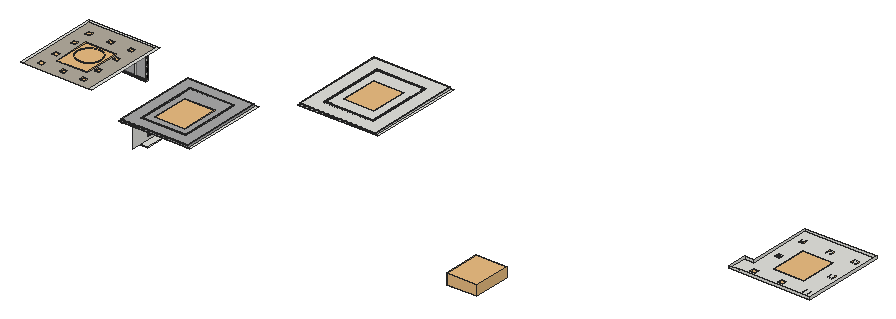
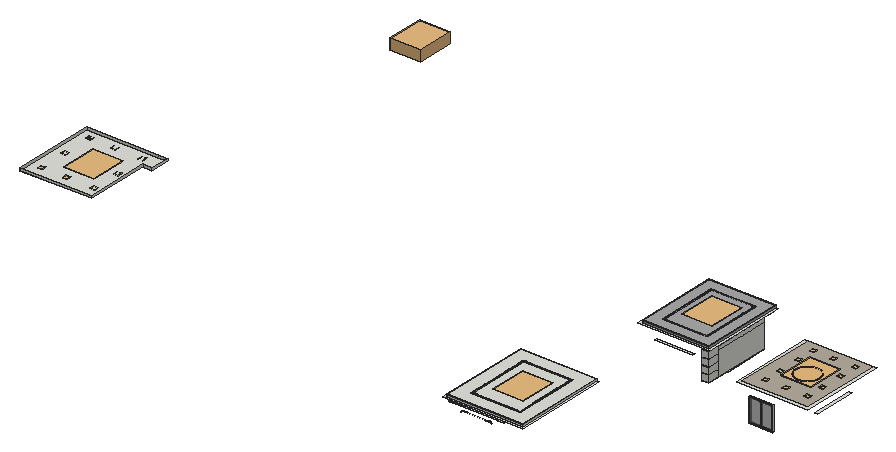
# SketchUp Ruby script. Lengths in inches.
U = 1.inch
M = Sketchup.active_model
def pt(a) = Geom::Point3d.new(a.map { |v| v * U })
def face(e, loops, mat)
  f = e.add_face(loops[0].map { |a| pt(a) })
  loops[1..].each { |l| e.add_face(l.map { |a| pt(a) }).erase! }
  f.material = f.back_material = mat if mat
  f
end
# faces: each face lists its corners as indices into pts; further lists are holes
def faces(e, pts, list, mat = nil) = list.each { |f| face(e, (f[0].is_a?(Array) ? f : [f]).map { |l| l.map { |i| pts[i] } }, mat) }
# xy, xz, yz: faces in a plane at the given z, y or x. An outline is a flat list of corners, or four numbers for a rectangle; further outlines are holes
def ring(l) = l.size == 4 ? [[l[0], l[1]], [l[2], l[1]], [l[2], l[3]], [l[0], l[3]]] : l.each_slice(2).to_a
def flat(e, list, mat, &to3) = list.each { |f| face(e, (f[0].is_a?(Array) ? f : [f]).map { |l| ring(l).map { |u, v| to3.(u, v) } }, mat) }
def xy(e, z, list, mat = nil) = flat(e, list, mat) { |x, y| [x, y, z] }
def xz(e, y, list, mat = nil) = flat(e, list, mat) { |x, z| [x, y, z] }
def yz(e, x, list, mat = nil) = flat(e, list, mat) { |y, z| [x, y, z] }
def lines(e, pts, list) = list.each { |a, b| e.add_line(pt(pts[a]), pt(pts[b])) }
# prism: a flat outline (further loops are holes) pulled along v
def prism(e, loops, v, mat = nil)
  f = face(e, loops, mat); d = Geom::Vector3d.new(v.map { |x| x * U })
  f.pushpull(f.normal.samedirection?(d) ? d.length : -d.length)
end
def box(e, o, s, mat = nil) = prism(e, [[o, [o[0] + s[0], o[1], o[2]], [o[0] + s[0], o[1] + s[1], o[2]], [o[0], o[1] + s[1], o[2]]]], [0, 0, s[2]], mat)
def at(x, y, z, deg = 0) = Geom::Transformation.translation(pt([x, y, z])) * Geom::Transformation.rotation(ORIGIN, Z_AXIS, deg.degrees)
def axes(o, x, y, z) = Geom::Transformation.new([*x, 0, *y, 0, *z, 0, *pt(o).to_a, 1])
def part(name) = M.definitions.add(name)
# library, detail: a bought-in or finely detailed component or shape, given as its bounding box
def library(name, o, s) = part(name).tap { |d| box(d.entities, o, s) }
def detail(e, o, s) = box(e.add_group.entities, o, s)
def put(e, d, t, mat = nil) = e.add_instance(d, t).tap { |i| i.material = mat if mat }
def group(e, t, mat = nil) = e.add_group.tap { |g| g.transformation = t; g.material = mat if mat }.entities
root = M.entities
M.materials.add("[0136_Charcoal]").color = [35, 35, 35]
M.materials.add("[Color M03]").color = [170, 170, 170]
M.materials.add("[Color_008]").color = [30, 30, 30]
M.materials.add("[Color_009]").color = [0, 0, 0]
M.materials.add("[Color_B19]").color = [180, 172, 158]
M.materials.add("[Translucent_Glass_Gray]").color = [128, 128, 128]
M.materials["[Translucent_Glass_Gray]"].alpha = 0.5
c1 = library("ceiling fan",[0,0,0],[76.25,93.13,30.02])
c2 = part("Enscape.LinearLight\#3")
xz(c2.entities,-55.62,[[0,-1,0,0,-0.38,-0.92],[0,-1,0.38,-0.92,0,0],[-0.38,-0.92,0,0,-0.71,-0.71],[0.38,-0.92,0.71,-0.71,0,0],[-0.71,-0.71,0,0,-0.92,-0.38],
  [0.71,-0.71,0.92,-0.38,0,0],[-0.92,-0.38,0,0,-1,0],[0.92,-0.38,1,0,0,0],[-1,0,0,0,-0.92,0.38],[0,0,-0.71,0.71,-0.92,0.38],
  [0,0,-0.38,0.92,-0.71,0.71],[0,0,0,1,-0.38,0.92],[0,0,0.38,0.92,0,1],[0,0,0.71,0.71,0.38,0.92],[0,0,0.92,0.38,0.71,0.71],
  [0,0,1,0,0.92,0.38]])
xz(c2.entities,55.62,[[0,-1,-0.38,-0.92,0,0],[0,-1,0,0,0.38,-0.92],[-0.38,-0.92,-0.71,-0.71,0,0],[0.38,-0.92,0,0,0.71,-0.71],[-0.71,-0.71,-0.92,-0.38,0,0],
  [0.71,-0.71,0,0,0.92,-0.38],[-0.92,-0.38,-1,0,0,0],[0.92,-0.38,0,0,1,0],[-1,0,-0.92,0.38,0,0],[0,0,-0.92,0.38,-0.71,0.71],
  [0,0,-0.71,0.71,-0.38,0.92],[0,0,-0.38,0.92,0,1],[0,0,0,1,0.38,0.92],[0,0,0.38,0.92,0.71,0.71],[0,0,0.71,0.71,0.92,0.38],
  [0,0,0.92,0.38,1,0]])
p = [[-0.38,-55.62,-0.92],[-0.38,55.62,-0.92],[0,55.62,-1],[0,-55.62,-1],[0.38,55.62,-0.92],[0.38,-55.62,-0.92],
  [-0.71,-55.62,-0.71],[-0.71,55.62,-0.71],[0.71,55.62,-0.71],[0.71,-55.62,-0.71],[-0.92,-55.62,-0.38],[-0.92,55.62,-0.38],
  [0.92,55.62,-0.38],[0.92,-55.62,-0.38],[-1,-55.62,0],[-1,55.62,0],[1,55.62,0],[1,-55.62,0],
  [-0.92,-55.62,0.38],[-0.92,55.62,0.38],[0.92,55.62,0.38],[0.92,-55.62,0.38],[-0.71,-55.62,0.71],[-0.71,55.62,0.71],
  [0.71,55.62,0.71],[0.71,-55.62,0.71],[-0.38,-55.62,0.92],[-0.38,55.62,0.92],[0.38,55.62,0.92],[0.38,-55.62,0.92],
  [0,-55.62,1],[0,55.62,1]]
faces(c2.entities,p,[[0,1,2],[0,2,3],[3,2,4],[3,4,5],[6,7,1],[6,1,0],[5,4,8],[5,8,9],
  [10,11,7],[10,7,6],[9,8,12],[9,12,13],[14,15,11],[14,11,10],[13,12,16],[13,16,17],
  [18,19,15],[18,15,14],[17,16,20],[17,20,21],[22,23,19],[22,19,18],[21,20,24],[21,24,25],
  [26,27,23],[26,23,22],[25,24,28],[25,28,29],[30,31,27],[30,27,26],[29,28,31],[29,31,30]])
c3 = part("Group\#24")
put(c3.entities,c2,at(55.62,1,1,-90))
put(c3.entities,c2,at(64.38,1,1,-90))
c4 = part("Group\#25")
put(c4.entities,c3,at(2,0,0,90))
put(c4.entities,c3,at(2,42,0,90))
c5 = library("Group\#26",[-1.6,-2.28,-0.2],[11.2,11.87,10.47])
c6 = library("Group\#11",[-1.89,-1.55,0],[10.94,10.95,9.68])
c7 = part("Enscape.LinearLight")
xz(c7.entities,-59.06,[[0,-1,0,0,-0.38,-0.92],[0,-1,0.38,-0.92,0,0],[-0.38,-0.92,0,0,-0.71,-0.71],[0.38,-0.92,0.71,-0.71,0,0],[-0.71,-0.71,0,0,-0.92,-0.38],
  [0.71,-0.71,0.92,-0.38,0,0],[-0.92,-0.38,0,0,-1,0],[0.92,-0.38,1,0,0,0],[-1,0,0,0,-0.92,0.38],[0,0,-0.71,0.71,-0.92,0.38],
  [0,0,-0.38,0.92,-0.71,0.71],[0,0,0,1,-0.38,0.92],[0,0,0.38,0.92,0,1],[0,0,0.71,0.71,0.38,0.92],[0,0,0.92,0.38,0.71,0.71],
  [0,0,1,0,0.92,0.38]])
xz(c7.entities,59.06,[[0,-1,-0.38,-0.92,0,0],[0,-1,0,0,0.38,-0.92],[-0.38,-0.92,-0.71,-0.71,0,0],[0.38,-0.92,0,0,0.71,-0.71],[-0.71,-0.71,-0.92,-0.38,0,0],
  [0.71,-0.71,0,0,0.92,-0.38],[-0.92,-0.38,-1,0,0,0],[0.92,-0.38,0,0,1,0],[-1,0,-0.92,0.38,0,0],[0,0,-0.92,0.38,-0.71,0.71],
  [0,0,-0.71,0.71,-0.38,0.92],[0,0,-0.38,0.92,0,1],[0,0,0,1,0.38,0.92],[0,0,0.38,0.92,0.71,0.71],[0,0,0.71,0.71,0.92,0.38],
  [0,0,0.92,0.38,1,0]])
p = [[-0.38,-59.06,-0.92],[-0.38,59.06,-0.92],[0,59.06,-1],[0,-59.06,-1],[0.38,59.06,-0.92],[0.38,-59.06,-0.92],
  [-0.71,-59.06,-0.71],[-0.71,59.06,-0.71],[0.71,59.06,-0.71],[0.71,-59.06,-0.71],[-0.92,-59.06,-0.38],[-0.92,59.06,-0.38],
  [0.92,59.06,-0.38],[0.92,-59.06,-0.38],[-1,-59.06,0],[-1,59.06,0],[1,59.06,0],[1,-59.06,0],
  [-0.92,-59.06,0.38],[-0.92,59.06,0.38],[0.92,59.06,0.38],[0.92,-59.06,0.38],[-0.71,-59.06,0.71],[-0.71,59.06,0.71],
  [0.71,59.06,0.71],[0.71,-59.06,0.71],[-0.38,-59.06,0.92],[-0.38,59.06,0.92],[0.38,59.06,0.92],[0.38,-59.06,0.92],
  [0,-59.06,1],[0,59.06,1]]
faces(c7.entities,p,[[0,1,2],[0,2,3],[3,2,4],[3,4,5],[6,7,1],[6,1,0],[5,4,8],[5,8,9],
  [10,11,7],[10,7,6],[9,8,12],[9,12,13],[14,15,11],[14,11,10],[13,12,16],[13,16,17],
  [18,19,15],[18,15,14],[17,16,20],[17,20,21],[22,23,19],[22,19,18],[21,20,24],[21,24,25],
  [26,27,23],[26,23,22],[25,24,28],[25,28,29],[30,31,27],[30,27,26],[29,28,31],[29,31,30]])
c8 = part("Group\#9")
put(c8.entities,c7,at(1,59.06,1))
put(c8.entities,c7,at(1,90.94,1))
c9 = library("Group\#10",[0,0,0],[108,2,2])
c10 = library("Group\#53",[-1.63,-0.87,0],[11.47,11.27,10.08])
c11 = library("Group\#40",[-1.73,-1.35,-0.07],[10.56,10.17,9.31])
xy(root,36,[[90,610.17,150,616.17]])
xy(root,37.6,[[555.98,931.54,615.33,932.04]])
xy(root,40,[[305.13,399.45,323.13,485.45]])
xy(root,41.5,[[305.13,518.45,323.13,546.45]])
xy(root,42,[[305.13,373.45,306.13,397.45],[306.13,397.45,323.13,487.45],[305.13,487.45,306.13,517.45]])
xy(root,42.5,[[305.13,518.45,323.13,546.45]])
xy(root,46.35,[[515.52,920.04,531.52,932.04],[637.52,920.04,653.52,932.04]])
xy(root,47.35,[[524.52,914.04,523.22,914.12,521.93,914.375,520.69,914.8,519.52,915.375,518.43,916.1,517.45,916.97,516.59,917.95,515.86,919.04,515.37,920.04,532.52,920.04,532.52,914.04],[532.52,914.04,533.52,932.04],[533.52,914.04,636.52,932.04],[636.52,914.04,636.52,920.04,653.67,920.04,653.18,919.04,652.45,917.95,651.59,916.97,650.61,916.1,649.52,915.375,648.35,914.8,647.11,914.375,645.83,914.12,644.52,914.04],[514.52,920.04,515.37,920.04,515.28,920.21,514.86,921.45,514.61,922.73,514.52,924.04],
  [653.67,920.04,654.52,920.04,654.52,924.04,654.4375,922.73,654.18,921.45,653.76,920.21]])
xy(root,51.35,[[524.52,914.04,644.52,914.04,645.83,914.12,647.11,914.375,648.35,914.8,649.52,915.375,650.61,916.1,651.59,916.97,652.45,917.95,653.18,919.04,653.76,920.21,654.18,921.45,654.4375,922.73,654.52,924.04,654.52,932.04,514.52,932.04,514.52,924.04,514.61,922.73,514.86,921.45,515.28,920.21,515.86,919.04,516.59,917.95,517.45,916.97,518.43,916.1,519.52,915.375,520.69,914.8,521.93,914.375,523.22,914.12]])
xy(root,55.35,[[462.52,698.04,468.52,698.04,468.52,932.04,660.52,932.04,660.52,698.04,666.52,698.04,666.52,938.04,462.52,938.04]])
xy(root,59.25,[[305.13,518.45,323.13,546.45]])
xy(root,60.25,[[305.13,518.45,323.13,546.45]])
xy(root,77,[[305.13,518.45,323.13,546.45]])
xy(root,78,[[305.13,518.45,323.13,546.45]])
xy(root,94.75,[[305.13,518.45,323.13,546.45]])
xy(root,95.75,[[305.13,518.45,323.13,546.45]])
xy(root,96,[[0,478.17,6,586.17],[341.13,547.45,437.13,553.45],[90,610.17,150,616.17]])
xy(root,113,[[305.13,518.45,323.13,546.45]])
xy(root,114,[[305.13,373.45,306.13,517.45],[305.13,517.45,323.13,547.45]])
xy(root,120,[[299.13,337.45,305.13,337.45,305.13,547.45,473.13,547.45,473.13,337.45,479.13,337.45,479.13,553.45,299.13,553.45],[0,400.17,6,400.17,6,610.17,174,610.17,174,400.17,180,400.17,180,616.17,0,616.17]])
xz(root,373.45,[[305.13,42,306.13,114]])
xz(root,517.45,[[306.13,42,323.13,114]])
xz(root,518.45,[[305.13,42.5,323.13,59.25],[305.13,60.25,323.13,77],[305.13,78,323.13,94.75],[305.13,95.75,323.13,113]])
xz(root,546.45,[[305.13,42.5,323.13,59.25],[305.13,60.25,323.13,77],[305.13,78,323.13,94.75],[305.13,95.75,323.13,113]])
xz(root,914.04,[[524.52,47.35,644.52,51.35]])
yz(root,90,[[610.17,36,616.17,96]])
yz(root,150,[[610.17,36,616.17,96]])
yz(root,305.13,[[518.45,42.5,546.45,59.25],[518.45,60.25,546.45,77],[518.45,78,546.45,94.75],[518.45,95.75,546.45,113]])
yz(root,306.13,[[373.45,42,517.45,102],[373.45,102,517.45,114]])
yz(root,323.13,[[518.45,41.5,546.45,42.5],[518.45,59.25,546.45,60.25],[518.45,77,546.45,78],[518.45,94.75,546.45,95.75]])
yz(root,514.52,[[924.04,47.35,932.04,51.35]])
yz(root,654.52,[[924.04,47.35,932.04,51.35]])
p = [[547.49,932.04,34.09],[546.46,932.04,32.91],[546.46,931.54,32.91],[547.49,931.54,34.09],[624.85,932.04,32.91],[623.82,932.04,34.09],
  [623.82,931.54,34.09],[624.85,931.54,32.91],[548.67,932.04,35.125],[548.67,931.54,35.125],[622.64,932.04,35.125],[622.64,931.54,35.125],
  [549.98,932.04,36],[549.98,931.54,36],[621.33,932.04,36],[621.33,931.54,36],[551.39,932.04,36.69],[551.39,931.54,36.69],
  [619.93,932.04,36.69],[619.93,931.54,36.69],[552.875,932.04,37.2],[552.875,931.54,37.2],[618.4375,932.04,37.2],[618.4375,931.54,37.2],
  [554.41,932.04,37.5],[554.41,931.54,37.5],[616.9,932.04,37.5],[616.9,931.54,37.5],[555.98,932.04,37.6],[555.98,931.54,37.6],
  [615.33,932.04,37.6],[615.33,931.54,37.6],[524.52,914.04,51.35],[523.22,914.12,51.35],[523.22,914.12,47.35],[524.52,914.04,47.35],
  [645.83,914.12,51.35],[644.52,914.04,51.35],[644.52,914.04,47.35],[645.83,914.12,47.35],[521.93,914.375,51.35],[521.93,914.375,47.35],
  [647.11,914.375,51.35],[647.11,914.375,47.35],[520.69,914.8,51.35],[520.69,914.8,47.35],[648.35,914.8,51.35],[648.35,914.8,47.35],
  [519.52,915.375,51.35],[519.52,915.375,47.35],[649.52,915.375,51.35],[649.52,915.375,47.35],[518.43,916.1,51.35],[518.43,916.1,47.35],
  [650.61,916.1,51.35],[650.61,916.1,47.35],[517.45,916.97,51.35],[517.45,916.97,47.35],[651.59,916.97,51.35],[651.59,916.97,47.35],
  [516.59,917.95,51.35],[516.59,917.95,47.35],[652.45,917.95,51.35],[652.45,917.95,47.35],[515.86,919.04,51.35],[515.86,919.04,47.35],
  [653.18,919.04,51.35],[653.18,919.04,47.35],[515.28,920.21,51.35],[515.28,920.21,47.35],[515.37,920.04,47.35],[653.76,920.21,51.35],
  [653.67,920.04,47.35],[653.76,920.21,47.35],[514.86,921.45,51.35],[514.86,921.45,47.35],[654.18,921.45,51.35],[654.18,921.45,47.35],
  [514.61,922.73,51.35],[514.61,922.73,47.35],[654.4375,922.73,51.35],[654.4375,922.73,47.35],[514.52,924.04,51.35],[514.52,924.04,47.35],
  [654.52,924.04,51.35],[654.52,924.04,47.35],[305.13,373.45,114],[305.13,338.45,114]]
faces(root,p,[[0,1,2,3],[4,5,6,7],[8,0,3,9],[5,10,11,6],[12,8,9,13],[10,14,15,11],[16,12,13,17],[14,18,19,15],
  [20,16,17,21],[18,22,23,19],[24,20,21,25],[22,26,27,23],[28,24,25,29],[26,30,31,27],[32,33,34,35],[36,37,38,39],
  [33,40,41,34],[42,36,39,43],[40,44,45,41],[46,42,43,47],[44,48,49,45],[50,46,47,51],[48,52,53,49],[54,50,51,55],
  [52,56,57,53],[58,54,55,59],[56,60,61,57],[62,58,59,63],[60,64,65,61],[66,62,63,67],[64,68,69,70,65],[71,66,67,72,73],
  [68,74,75,69],[76,71,73,77],[74,78,79,75],[80,76,77,81],[78,82,83,79],[84,80,81,85]])
lines(root,p,[[86,87]])
g1 = group(root,at(90,612.37,36))
xy(g1,0,[[0,0,60,2.22]],"[Color_009]")
xy(g1,1.43,[[1.43,1.85,29.29,2.22],[30.71,1.85,58.57,2.22]])
xy(g1,1.43,[[1.43,0,29.29,0.56],[30.71,0,58.57,0.56]],"[Color_009]")
xy(g1,58.57,[[1.43,0,29.29,0.56],[30.71,0,58.57,0.56],[1.43,0.56,29.29,1.85],[30.71,0.56,58.57,1.85],[1.43,1.85,29.29,2.22],
  [30.71,1.85,58.57,2.22]])
xy(g1,60,[[0,0,60,2.22]],"[Color_008]")
xz(g1,0,[[[0,0,60,60],[1.43,1.43,29.29,58.57],[30.71,1.43,58.57,58.57]]],"[Color_009]")
xz(g1,0.56,[[1.43,1.43,29.29,58.57],[30.71,1.43,58.57,58.57]],"[Translucent_Glass_Gray]")
xz(g1,1.85,[[1.43,1.43,29.29,58.57],[30.71,1.43,58.57,58.57]],"[Translucent_Glass_Gray]")
xz(g1,2.22,[[[0,0,60,60],[1.43,1.43,58.57,58.57]],[29.29,1.43,30.71,58.57]],"[Color_009]")
yz(g1,0,[[0,0,2.22,60]],"[Color_009]")
yz(g1,1.43,[[1.85,1.43,2.22,58.57]])
yz(g1,1.43,[[0,1.43,0.56,58.57]],"[Color_009]")
yz(g1,29.29,[[0,1.43,0.56,58.57],[1.85,1.43,2.22,58.57]],"[Color_009]")
yz(g1,30.71,[[0,1.43,0.56,58.57],[1.85,1.43,2.22,58.57]])
yz(g1,58.57,[[0,1.43,0.56,58.57],[1.85,1.43,2.22,58.57]],"[Color_009]")
yz(g1,60,[[0,0,2.22,60]],"[Color_009]")
put(root,c1,axes([526.02,765.21,36.44],[1,0,0],[0,1,0],[0,0,0.83]))
g2 = group(root,at(468.52,698.04,61.35))
xy(g2,-6,[[[0,0,192,234],[36,36,156,198]]])
xy(g2,-2,[[[0,0,192,234],[34,34,158,200]],[34,34,36,200],[36,34,156,36],[156,34,158,200],[36,198,156,200]])
xy(g2,0,[[[0,0,192,234],[34,34,158,200]],[34,34,158,200]])
xz(g2,0,[[0,-6,192,-2],[0,-2,192,0]])
xz(g2,34,[[34,-2,158,0]])
xz(g2,36,[[36,-6,156,-2]])
xz(g2,198,[[36,-6,156,-2]])
xz(g2,200,[[34,-2,158,0]])
xz(g2,234,[[0,-6,192,-2],[0,-2,192,0]])
yz(g2,0,[[0,-6,234,-2],[0,-2,234,0]])
yz(g2,34,[[34,-2,200,0]])
yz(g2,36,[[36,-6,198,-2]])
yz(g2,156,[[36,-6,198,-2]])
yz(g2,158,[[34,-2,200,0]])
yz(g2,192,[[0,-6,234,-2],[0,-2,234,0]])
put(g2,c3,at(36,34,-2))
put(g2,c3,at(36,197.71,-2.11))
put(g2,c4,at(34,36,-2))
put(g2,c4,at(156,36,-2))
put(g2,c5,axes([27.0625,210.32,-6],[-1,0,0],[0,1,0],[0,0,-1]))
put(g2,c5,axes([27.0625,18.01,-6],[-1,0,0],[0,1,0],[0,0,-1]))
put(g2,c5,axes([27.0625,152.76,-6],[-1,0,0],[0,1,0],[0,0,-1]))
put(g2,c5,axes([27.0625,84.88,-6],[-1,0,0],[0,1,0],[0,0,-1]))
put(g2,c5,axes([177.25,210.32,-6],[-1,0,0],[0,1,0],[0,0,-1]))
put(g2,c5,axes([177.25,18.01,-6],[-1,0,0],[0,1,0],[0,0,-1]))
put(g2,c5,axes([177.25,84.88,-6],[-1,0,0],[0,1,0],[0,0,-1]))
put(g2,c5,axes([177.25,152.76,-6],[-1,0,0],[0,1,0],[0,0,-1]))
put(g2,c5,axes([127.75,210.32,-6],[-1,0,0],[0,1,0],[0,0,-1]))
put(g2,c5,axes([127.75,18.01,-6],[-1,0,0],[0,1,0],[0,0,-1]))
put(g2,c5,axes([74.875,18.01,-6],[-1,0,0],[0,1,0],[0,0,-1]))
put(g2,c5,axes([74.875,210.32,-6],[-1,0,0],[0,1,0],[0,0,-1]))
g3 = group(root,at(316.68,475.54,57.94),"[0136_Charcoal]")
xy(g3,0,[[-2,-64.62,0,0]])
xy(g3,16.76,[[-5,-36.94,-2,-25.88]])
xy(g3,22.39,[[-5,-36.94,-2,-25.88]])
xy(g3,39.9375,[[-2,-64.62,0,0]])
xz(g3,-64.62,[[-2,0,0,39.9375]])
xz(g3,-36.94,[[-5,16.76,-2,22.39]])
xz(g3,-25.88,[[-5,16.76,-2,22.39]])
xz(g3,0,[[-2,0,0,39.9375]])
yz(g3,-5,[[-36.94,16.76,-25.88,22.39]])
yz(g3,-2,[[[-64.62,0,0,39.9375],[-36.94,16.76,-25.88,22.39]]])
yz(g3,0,[[-64.62,0,0,39.9375]])
put(root,c1,at(52.03,449.6,89.92))
put(root,c1,axes([1681.09,677.99,93.89],[1,0,0],[0,1,0],[0,0,0.87]))
g4 = group(root,at(305.13,337.45,99.59))
put(g4,c1,axes([46.47,48.28,0],[1,0,0],[0,1,0],[0,0,0.88]))
put(g4,c1,axes([1039.46,-270.54,134.97],[1,0,0],[0,1,0],[0,0,0.88]))
g5 = group(g4,at(0,0,26.41),"[Color M03]")
xy(g5,-6,[[[0,0,168,210],[30,30,138,180]]])
xy(g5,-2,[[[0,0,168,210],[28,28,140.0625,182]],[28,28,30,182],[30,28,138,30],[138,28,140.0625,180],[30,180,140.0625,182]])
xy(g5,0,[[[0,0,168,210],[28,28,140.0625,182]],[28,28,140.0625,182]])
xz(g5,0,[[0,-6,168,-2],[0,-2,168,0]])
xz(g5,28,[[28,-2,140.0625,0]])
xz(g5,30,[[30,-6,138,-2]])
xz(g5,180,[[30,-6,138,-2]])
xz(g5,182,[[28,-2,140.0625,0]])
xz(g5,210,[[0,-6,168,-2],[0,-2,168,0]])
yz(g5,0,[[0,-6,210,-2],[0,-2,210,0]])
yz(g5,28,[[28,-2,182,0]])
yz(g5,30,[[30,-6,180,-2]])
yz(g5,138,[[30,-6,180,-2]])
yz(g5,140.0625,[[28,-2,182,0]])
yz(g5,168,[[0,-6,210,-2],[0,-2,210,0]])
put(g5,c6,axes([21.93,188.33,-6],[-1,0,0],[0,1,0],[0,0,-1]))
put(g5,c6,axes([21.93,13.7,-6],[-1,0,0],[0,1,0],[0,0,-1]))
put(g5,c6,axes([21.93,135.45,-6],[-1,0,0],[0,1,0],[0,0,-1]))
put(g5,c6,axes([21.93,75.58,-6],[-1,0,0],[0,1,0],[0,0,-1]))
put(g5,c6,axes([154.87,135.45,-6],[-1,0,0],[0,1,0],[0,0,-1]))
put(g5,c6,axes([154.87,188.33,-6],[-1,0,0],[0,1,0],[0,0,-1]))
put(g5,c6,axes([154.87,13.7,-6],[-1,0,0],[0,1,0],[0,0,-1]))
put(g5,c6,axes([154.87,75.58,-6],[-1,0,0],[0,1,0],[0,0,-1]))
put(g5,c6,axes([86.49,188.33,-6],[-1,0,0],[0,1,0],[0,0,-1]))
put(g5,c6,axes([86.49,13.7,-6],[-1,0,0],[0,1,0],[0,0,-1]))
put(g4,c8,at(28,30,24.41))
put(g4,c8,at(138,30,24.41))
put(g4,c9,at(30,28,24.41))
put(g4,c9,at(30,179.6875,24.04))
g6 = group(root,at(1635.15,625.74,126))
xy(g6,-6,[[-24,0,-24,48,0,48,0,210,180,210,180,0]])
xz(g6,0,[[-24,-6,0,0],[0,-6,180,0]])
xz(g6,48,[[-24,-6,0,0]])
xz(g6,210,[[0,-6,180,0]])
yz(g6,-24,[[0,-6,48,0]])
yz(g6,0,[[48,-6,210,0]])
yz(g6,180,[[0,-6,210,0]])
put(g6,c10,axes([26.07,17.24,-6],[-1,0,0],[0,1,0],[0,0,-1]))
put(g6,c10,axes([159.26,17.24,-6],[-1,0,0],[0,1,0],[0,0,-1]))
put(g6,c10,axes([159.26,169.74,-6],[-1,0,0],[0,1,0],[0,0,-1]))
put(g6,c10,axes([26.07,169.74,-6],[-1,0,0],[0,1,0],[0,0,-1]))
put(g6,c10,axes([159.26,95.12,-6],[-1,0,0],[0,1,0],[0,0,-1]))
put(g6,c10,axes([26.07,95.12,-6],[-1,0,0],[0,1,0],[0,0,-1]))
put(g6,c10,axes([95.88,169.74,-6],[-1,0,0],[0,1,0],[0,0,-1]))
put(g6,c10,axes([95.88,17.24,-6],[-1,0,0],[0,1,0],[0,0,-1]))
g7 = group(root,at(6,400.17,119.93),"[Color_B19]")
xy(g7,-6,[[83.51,75,81.625,75.09,79.75,75.3,77.9,75.63,76.0625,76.07,74.26,76.625,72.5,77.29,70.78,78.07,69.12,78.95,67.51,79.9375,65.97,81.02,64.5,82.2,63.11,83.47,61.8,84.83,60.57,86.26,59.44,87.77,58.41,89.34,57.48,90.98,56.65,92.67,55.93,94.42,55.32,96.2,54.82,98.02,54.44,99.86,54.18,101.73,54.03,103.61,54,105.49,54.09,107.375,54.3,109.25,54.63,111.1,55.07,112.9375,55.625,114.74,56.29,116.5,57.07,118.22,57.95,119.88,58.9375,121.49,60.02,123.03,61.2,124.5,62.47,125.89,63.83,127.2,65.26,128.43,66.77,129.56,68.34,130.59,69.98,131.52,71.67,132.35,73.42,133.07,75.2,133.68,77.02,134.18,78.86,134.56,80.73,134.82,82.61,134.97,84.49,135,86.375,134.91,88.25,134.7,90.1,134.37,91.9375,133.93,93.74,133.375,95.5,132.71,97.22,131.93,98.88,131.05,100.49,130.0625,102.03,128.98,103.5,127.8,104.89,126.53,106.2,125.17,107.43,123.74,108.56,122.23,109.59,120.66,110.52,119.02,111.35,117.33,112.07,115.58,112.68,113.8,113.18,111.98,113.56,110.14,113.82,108.27,113.97,106.39,114,104.51,113.91,102.625,113.7,100.75,113.37,98.9,112.93,97.0625,112.375,95.26,111.71,93.5,110.93,91.78,110.05,90.12,109.0625,88.51,107.98,86.97,106.8,85.5,105.53,84.11,104.17,82.8,102.74,81.57,101.23,80.44,99.66,79.41,98.02,78.48,96.33,77.65,94.58,76.93,92.8,76.32,90.98,75.82,89.14,75.44,87.27,75.18,85.39,75.03]])
xy(g7,0,[[[0,0,168,210],[83.51,75,85.39,75.03,87.27,75.18,89.14,75.44,90.98,75.82,92.8,76.32,94.58,76.93,96.33,77.65,98.02,78.48,99.66,79.41,101.23,80.44,102.74,81.57,104.17,82.8,105.53,84.11,106.8,85.5,107.98,86.97,109.0625,88.51,110.05,90.12,110.93,91.78,111.71,93.5,112.375,95.26,112.93,97.0625,113.37,98.9,113.7,100.75,113.91,102.625,114,104.51,113.97,106.39,113.82,108.27,113.56,110.14,113.18,111.98,112.68,113.8,112.07,115.58,111.35,117.33,110.52,119.02,109.59,120.66,108.56,122.23,107.43,123.74,106.2,125.17,104.89,126.53,103.5,127.8,102.03,128.98,100.49,130.0625,98.88,131.05,97.22,131.93,95.5,132.71,93.74,133.375,91.9375,133.93,90.1,134.37,88.25,134.7,86.375,134.91,84.49,135,82.61,134.97,80.73,134.82,78.86,134.56,77.02,134.18,75.2,133.68,73.42,133.07,71.67,132.35,69.98,131.52,68.34,130.59,66.77,129.56,65.26,128.43,63.83,127.2,62.47,125.89,61.2,124.5,60.02,123.03,58.9375,121.49,57.95,119.88,57.07,118.22,56.29,116.5,55.625,114.74,55.07,112.9375,54.63,111.1,54.3,109.25,54.09,107.375,54,105.49,54.03,103.61,54.18,101.73,54.44,99.86,54.82,98.02,55.32,96.2,55.93,94.42,56.65,92.67,57.48,90.98,58.41,89.34,59.44,87.77,60.57,86.26,61.8,84.83,63.11,83.47,64.5,82.2,65.97,81.02,67.51,79.9375,69.12,78.95,70.78,78.07,72.5,77.29,74.26,76.625,76.0625,76.07,77.9,75.63,79.75,75.3,81.625,75.09]]])
p = [[83.51,75,0],[81.625,75.09,0],[81.625,75.09,-6],[83.51,75,-6],[85.39,75.03,0],[85.39,75.03,-6],
  [87.27,75.18,0],[87.27,75.18,-6],[79.75,75.3,0],[79.75,75.3,-6],[89.14,75.44,0],[89.14,75.44,-6],
  [77.9,75.63,0],[77.9,75.63,-6],[90.98,75.82,0],[90.98,75.82,-6],[76.0625,76.07,0],[76.0625,76.07,-6],
  [92.8,76.32,0],[92.8,76.32,-6],[74.26,76.625,0],[74.26,76.625,-6],[94.58,76.93,0],[94.58,76.93,-6],
  [72.5,77.29,0],[72.5,77.29,-6],[96.33,77.65,0],[96.33,77.65,-6],[70.78,78.07,0],[70.78,78.07,-6],
  [98.02,78.48,0],[98.02,78.48,-6],[69.12,78.95,0],[69.12,78.95,-6],[99.66,79.41,0],[99.66,79.41,-6],
  [67.51,79.9375,0],[67.51,79.9375,-6],[101.23,80.44,0],[101.23,80.44,-6],[65.97,81.02,0],[65.97,81.02,-6],
  [102.74,81.57,0],[102.74,81.57,-6],[64.5,82.2,0],[64.5,82.2,-6],[104.17,82.8,0],[104.17,82.8,-6],
  [63.11,83.47,0],[63.11,83.47,-6],[105.53,84.11,0],[105.53,84.11,-6],[61.8,84.83,0],[61.8,84.83,-6],
  [106.8,85.5,0],[106.8,85.5,-6],[60.57,86.26,0],[60.57,86.26,-6],[107.98,86.97,0],[107.98,86.97,-6],
  [59.44,87.77,0],[59.44,87.77,-6],[109.0625,88.51,0],[109.0625,88.51,-6],[58.41,89.34,0],[58.41,89.34,-6],
  [110.05,90.12,0],[110.05,90.12,-6],[57.48,90.98,0],[57.48,90.98,-6],[110.93,91.78,0],[110.93,91.78,-6],
  [56.65,92.67,0],[56.65,92.67,-6],[111.71,93.5,0],[111.71,93.5,-6],[55.93,94.42,0],[55.93,94.42,-6],
  [112.375,95.26,0],[112.375,95.26,-6],[55.32,96.2,0],[55.32,96.2,-6],[112.93,97.0625,0],[112.93,97.0625,-6],
  [54.82,98.02,0],[54.82,98.02,-6],[113.37,98.9,0],[113.37,98.9,-6],[54.44,99.86,0],[54.44,99.86,-6],
  [113.7,100.75,0],[113.7,100.75,-6],[54.18,101.73,0],[54.18,101.73,-6],[113.91,102.625,0],[113.91,102.625,-6],
  [54.03,103.61,0],[54.03,103.61,-6],[114,104.51,0],[114,104.51,-6],[54,105.49,0],[54,105.49,-6],
  [113.97,106.39,0],[113.97,106.39,-6],[54.09,107.375,0],[54.09,107.375,-6],[113.82,108.27,0],[113.82,108.27,-6],
  [54.3,109.25,0],[54.3,109.25,-6],[113.56,110.14,0],[113.56,110.14,-6],[54.63,111.1,0],[54.63,111.1,-6],
  [113.18,111.98,0],[113.18,111.98,-6],[55.07,112.9375,0],[55.07,112.9375,-6],[112.68,113.8,0],[112.68,113.8,-6],
  [55.625,114.74,0],[55.625,114.74,-6],[112.07,115.58,0],[112.07,115.58,-6],[56.29,116.5,0],[56.29,116.5,-6],
  [111.35,117.33,0],[111.35,117.33,-6],[57.07,118.22,0],[57.07,118.22,-6],[110.52,119.02,0],[110.52,119.02,-6],
  [57.95,119.88,0],[57.95,119.88,-6],[109.59,120.66,0],[109.59,120.66,-6],[58.9375,121.49,0],[58.9375,121.49,-6],
  [108.56,122.23,0],[108.56,122.23,-6],[60.02,123.03,0],[60.02,123.03,-6],[107.43,123.74,0],[107.43,123.74,-6],
  [61.2,124.5,0],[61.2,124.5,-6],[106.2,125.17,0],[106.2,125.17,-6],[62.47,125.89,0],[62.47,125.89,-6],
  [104.89,126.53,0],[104.89,126.53,-6],[63.83,127.2,0],[63.83,127.2,-6],[103.5,127.8,0],[103.5,127.8,-6],
  [65.26,128.43,0],[65.26,128.43,-6],[102.03,128.98,0],[102.03,128.98,-6],[66.77,129.56,0],[66.77,129.56,-6],
  [100.49,130.0625,0],[100.49,130.0625,-6],[68.34,130.59,0],[68.34,130.59,-6],[98.88,131.05,0],[98.88,131.05,-6],
  [69.98,131.52,0],[69.98,131.52,-6],[97.22,131.93,0],[97.22,131.93,-6],[71.67,132.35,0],[71.67,132.35,-6],
  [95.5,132.71,0],[95.5,132.71,-6],[73.42,133.07,0],[73.42,133.07,-6],[93.74,133.375,0],[93.74,133.375,-6],
  [75.2,133.68,0],[75.2,133.68,-6],[91.9375,133.93,0],[91.9375,133.93,-6],[77.02,134.18,0],[77.02,134.18,-6],
  [90.1,134.37,0],[90.1,134.37,-6],[78.86,134.56,0],[78.86,134.56,-6],[88.25,134.7,0],[88.25,134.7,-6],
  [80.73,134.82,0],[80.73,134.82,-6],[86.375,134.91,0],[86.375,134.91,-6],[82.61,134.97,0],[82.61,134.97,-6],
  [84.49,135,0],[84.49,135,-6]]
faces(g7,p,[[0,1,2,3],[4,0,3,5],[6,4,5,7],[1,8,9,2],[10,6,7,11],[8,12,13,9],[14,10,11,15],[12,16,17,13],
  [18,14,15,19],[16,20,21,17],[22,18,19,23],[20,24,25,21],[26,22,23,27],[24,28,29,25],[30,26,27,31],[28,32,33,29],
  [34,30,31,35],[32,36,37,33],[38,34,35,39],[36,40,41,37],[42,38,39,43],[40,44,45,41],[46,42,43,47],[44,48,49,45],
  [50,46,47,51],[48,52,53,49],[54,50,51,55],[52,56,57,53],[58,54,55,59],[56,60,61,57],[62,58,59,63],[60,64,65,61],
  [66,62,63,67],[64,68,69,65],[70,66,67,71],[68,72,73,69],[74,70,71,75],[72,76,77,73],[78,74,75,79],[76,80,81,77],
  [82,78,79,83],[80,84,85,81],[86,82,83,87],[84,88,89,85],[90,86,87,91],[88,92,93,89],[94,90,91,95],[92,96,97,93],
  [98,94,95,99],[96,100,101,97],[102,98,99,103],[100,104,105,101],[106,102,103,107],[104,108,109,105],[110,106,107,111],[108,112,113,109],
  [114,110,111,115],[112,116,117,113],[118,114,115,119],[116,120,121,117],[122,118,119,123],[120,124,125,121],[126,122,123,127],[124,128,129,125],
  [130,126,127,131],[128,132,133,129],[134,130,131,135],[132,136,137,133],[138,134,135,139],[136,140,141,137],[142,138,139,143],[140,144,145,141],
  [146,142,143,147],[144,148,149,145],[150,146,147,151],[148,152,153,149],[154,150,151,155],[152,156,157,153],[158,154,155,159],[156,160,161,157],
  [162,158,159,163],[160,164,165,161],[166,162,163,167],[164,168,169,165],[170,166,167,171],[168,172,173,169],[174,170,171,175],[172,176,177,173],
  [178,174,175,179],[176,180,181,177],[182,178,179,183],[180,184,185,181],[186,182,183,187],[184,188,189,185],[190,186,187,191],[188,192,193,189],
  [194,190,191,195],[192,196,197,193],[198,194,195,199],[196,198,199,197]])
put(g7,c11,axes([31.75,20.1875,0],[-1,0,0],[0,1,0],[0,0,-1]))
put(g7,c11,axes([86.75,20.1875,0],[-1,0,0],[0,1,0],[0,0,-1]))
put(g7,c11,axes([138.18,20.1875,0],[-1,0,0],[0,1,0],[0,0,-1]))
put(g7,c11,axes([31.75,170.375,0],[-1,0,0],[0,1,0],[0,0,-1]))
put(g7,c11,axes([86.75,170.375,0],[-1,0,0],[0,1,0],[0,0,-1]))
put(g7,c11,axes([138.18,170.375,0],[-1,0,0],[0,1,0],[0,0,-1]))
put(g7,c11,axes([31.75,66.125,0],[-1,0,0],[0,1,0],[0,0,-1]))
put(g7,c11,axes([138.18,66.125,0],[-1,0,0],[0,1,0],[0,0,-1]))
put(g7,c11,axes([31.75,124.6875,0],[-1,0,0],[0,1,0],[0,0,-1]))
put(g7,c11,axes([138.18,124.6875,0],[-1,0,0],[0,1,0],[0,0,-1]))
